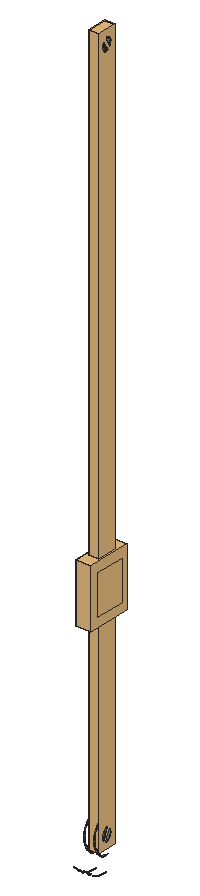
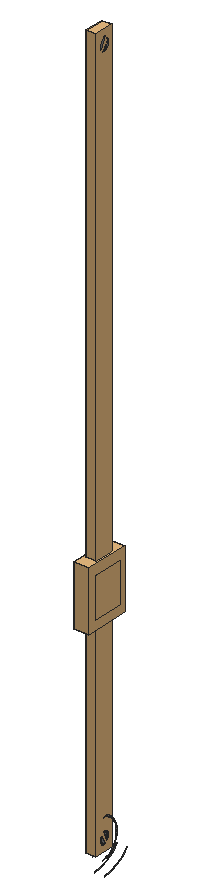
# SketchUp Ruby script. Lengths in inches.
U = 1.inch
M = Sketchup.active_model
def pt(a) = Geom::Point3d.new(a.map { |v| v * U })
def face(e, loops, mat)
  f = e.add_face(loops[0].map { |a| pt(a) })
  loops[1..].each { |l| e.add_face(l.map { |a| pt(a) }).erase! }
  f.material = f.back_material = mat if mat
  f
end
# faces: each face lists its corners as indices into pts; further lists are holes
def faces(e, pts, list, mat = nil) = list.each { |f| face(e, (f[0].is_a?(Array) ? f : [f]).map { |l| l.map { |i| pts[i] } }, mat) }
# xy, xz, yz: faces in a plane at the given z, y or x. An outline is a flat list of corners, or four numbers for a rectangle; further outlines are holes
def ring(l) = l.size == 4 ? [[l[0], l[1]], [l[2], l[1]], [l[2], l[3]], [l[0], l[3]]] : l.each_slice(2).to_a
def flat(e, list, mat, &to3) = list.each { |f| face(e, (f[0].is_a?(Array) ? f : [f]).map { |l| ring(l).map { |u, v| to3.(u, v) } }, mat) }
def xy(e, z, list, mat = nil) = flat(e, list, mat) { |x, y| [x, y, z] }
def xz(e, y, list, mat = nil) = flat(e, list, mat) { |x, z| [x, y, z] }
def yz(e, x, list, mat = nil) = flat(e, list, mat) { |y, z| [x, y, z] }
def lines(e, pts, list) = list.each { |a, b| e.add_line(pt(pts[a]), pt(pts[b])) }
# prism: a flat outline (further loops are holes) pulled along v
def prism(e, loops, v, mat = nil)
  f = face(e, loops, mat); d = Geom::Vector3d.new(v.map { |x| x * U })
  f.pushpull(f.normal.samedirection?(d) ? d.length : -d.length)
end
def box(e, o, s, mat = nil) = prism(e, [[o, [o[0] + s[0], o[1], o[2]], [o[0] + s[0], o[1] + s[1], o[2]], [o[0], o[1] + s[1], o[2]]]], [0, 0, s[2]], mat)
def at(x, y, z, deg = 0) = Geom::Transformation.translation(pt([x, y, z])) * Geom::Transformation.rotation(ORIGIN, Z_AXIS, deg.degrees)
def axes(o, x, y, z) = Geom::Transformation.new([*x, 0, *y, 0, *z, 0, *pt(o).to_a, 1])
def part(name) = M.definitions.add(name)
# library, detail: a bought-in or finely detailed component or shape, given as its bounding box
def library(name, o, s) = part(name).tap { |d| box(d.entities, o, s) }
def detail(e, o, s) = box(e.add_group.entities, o, s)
def put(e, d, t, mat = nil) = e.add_instance(d, t).tap { |i| i.material = mat if mat }
def group(e, t, mat = nil) = e.add_group.tap { |g| g.transformation = t; g.material = mat if mat }.entities
root = M.entities
M.materials.add("Material \#1").color = [140, 140, 140]
c1 = library("3DGeom~4_Defintion",[-18.02,-499.97,-221.16],[36.04,1000,262.12])
c2 = part("3DGeom~5_Defintion")
xy(c2.entities,-225.24,[[-0.79,-499.98,-2.33,-499.64,7.45,-496.14],[-0.79,-499.98,7.45,-496.14,1.58,-499.88],[1.58,-499.88,7.45,-496.14,3.84,-499.16],[-2.33,-499.64,7.4,-485.75,7.45,-496.14],[3.84,-499.16,7.45,-496.14,5.85,-497.89],
  [7.45,-496.14,7.4,-485.75,8.24,-487.08],[7.45,-496.14,8.24,-487.08,8.96,-489.34],[7.45,-496.14,8.96,-489.34,9.0625,-491.71],[7.45,-496.14,9.0625,-491.71,8.55,-494.03],[-7.4,-496.08,-8.24,-494.76,2.32,-482.2],
  [-8.24,-494.76,-8.96,-492.5,2.32,-482.2],[-8.96,-492.5,-9.0625,-490.125,2.32,-482.2],[-9.0625,-490.125,-8.55,-487.81,2.32,-482.2],[-8.55,-487.81,-7.45,-485.7,2.32,-482.2],[-7.45,-485.7,-5.85,-483.95,2.32,-482.2],
  [-5.85,-483.95,-3.84,-482.68,2.32,-482.2],[-3.84,-482.68,-1.58,-481.96,2.32,-482.2],[2.32,-482.2,-1.58,-481.96,0.79,-481.86],[0,481.82,-2.35,482.13,-6.92,496.71],[0,481.82,-6.92,496.71,1.55,482.04],
  [-2.35,482.13,-4.55,483.04,-6.92,496.71],[-4.55,483.04,-6.43,484.49,-6.92,496.71],[-6.43,484.49,-7.88,486.37,-6.92,496.71],[6.92,485.12,-1.55,499.8125,7.88,495.47],[6.92,485.12,7.88,495.47,7.88,486.37],
  [-7.88,486.37,-8.79,488.57,-6.92,496.71],[7.88,486.37,7.88,495.47,8.79,488.57],[-8.79,488.57,-9.1,490.92,-6.92,496.71],[8.79,488.57,7.88,495.47,9.1,490.92],[-9.1,490.92,-8.79,493.28,-6.92,496.71],
  [9.1,490.92,7.88,495.47,8.79,493.28],[-8.79,493.28,-7.88,495.47,-6.92,496.71],[7.88,495.47,-1.55,499.8125,0,500.02],[7.88,495.47,0,500.02,2.35,499.71],[7.88,495.47,2.35,499.71,4.55,498.8],
  [7.88,495.47,4.55,498.8,6.43,497.35]],"Material \#1")
xy(c2.entities,-221.57,[[-2.33,-499.64,-5.22,-498.37,7.4,-485.75],[-5.22,-498.37,-7.4,-496.08,5.22,-483.47],[-5.22,-498.37,5.22,-483.47,7.4,-485.75],[-7.4,-496.08,2.32,-482.2,5.22,-483.47],[1.55,482.04,-6.92,496.71,-4.55,498.8],
  [1.55,482.04,-4.55,498.8,4.55,483.04],[4.55,483.04,-4.55,498.8,-1.55,499.8125],[4.55,483.04,-1.55,499.8125,6.92,485.12]],"Material \#1")
xy(c2.entities,38.05,[[-2.33,-499.64,7.4,-485.75,-5.22,-498.37],[-5.22,-498.37,5.22,-483.47,-7.4,-496.08],[-5.22,-498.37,7.4,-485.75,5.22,-483.47],[-7.4,-496.08,5.22,-483.47,2.32,-482.2],[1.55,482.04,-4.55,498.8,-6.92,496.71],
  [1.55,482.04,4.55,483.04,-4.55,498.8],[4.55,483.04,-1.55,499.8125,-4.55,498.8],[4.55,483.04,6.92,485.12,-1.55,499.8125]],"Material \#1")
xy(c2.entities,41.72,[[-0.79,-499.98,7.45,-496.14,-2.33,-499.64],[-0.79,-499.98,1.58,-499.88,7.45,-496.14],[1.58,-499.88,3.84,-499.16,7.45,-496.14],[-2.33,-499.64,7.45,-496.14,7.4,-485.75],[3.84,-499.16,5.85,-497.89,7.45,-496.14],
  [7.45,-496.14,8.24,-487.08,7.4,-485.75],[7.45,-496.14,8.55,-494.03,9.0625,-491.71],[7.45,-496.14,8.96,-489.34,8.24,-487.08],[7.45,-496.14,9.0625,-491.71,8.96,-489.34],[-7.4,-496.08,2.32,-482.2,-8.24,-494.76],
  [-8.24,-494.76,2.32,-482.2,-8.96,-492.5],[-8.96,-492.5,2.32,-482.2,-9.0625,-490.125],[-9.0625,-490.125,2.32,-482.2,-8.55,-487.81],[-8.55,-487.81,2.32,-482.2,-7.45,-485.7],[-7.45,-485.7,2.32,-482.2,-5.85,-483.95],
  [-5.85,-483.95,2.32,-482.2,-3.84,-482.68],[-3.84,-482.68,2.32,-482.2,-1.58,-481.96],[2.32,-482.2,0.79,-481.86,-1.58,-481.96],[0,481.82,-6.92,496.71,-2.35,482.13],[0,481.82,1.55,482.04,-6.92,496.71],
  [-2.35,482.13,-6.92,496.71,-4.55,483.04],[-4.55,483.04,-6.92,496.71,-6.43,484.49],[-6.43,484.49,-6.92,496.71,-7.88,486.37],[6.92,485.12,7.88,495.47,-1.55,499.8125],[6.92,485.12,7.88,486.37,7.88,495.47],
  [-7.88,486.37,-6.92,496.71,-8.79,488.57],[7.88,486.37,8.79,488.57,7.88,495.47],[-8.79,488.57,-6.92,496.71,-9.1,490.92],[8.79,488.57,9.1,490.92,7.88,495.47],[-9.1,490.92,-6.92,496.71,-8.79,493.28],
  [9.1,490.92,8.79,493.28,7.88,495.47],[-8.79,493.28,-6.92,496.71,-7.88,495.47],[7.88,495.47,0,500.02,-1.55,499.8125],[7.88,495.47,2.35,499.71,0,500.02],[7.88,495.47,4.55,498.8,2.35,499.71],
  [7.88,495.47,6.43,497.35,4.55,498.8]],"Material \#1")
c3 = library("3DGeom~14_Defintion",[-102.17,352.37,-727.27],[204.35,204.35,1000])
c4 = library("3DGeom~1_Defintion",[-60.87,347.29,-704.08],[121.74,121.75,1000])
yz(root,263.952,[[328.177,50.586,328.059,50.6,328.061,50.614],[328.177,50.586,328.061,50.614,328.177,50.601],[328.059,50.6,327.948,50.64,327.952,50.654],[328.059,50.6,327.952,50.654,328.061,50.614],[327.948,50.64,327.846,50.704,327.852,50.717],
  [327.948,50.64,327.852,50.717,327.952,50.654],[327.846,50.704,327.762,50.801,327.852,50.717],[328.177,50.818,328.138,50.822,328.14,50.837],[328.177,50.818,328.14,50.837,328.177,50.832],[328.177,50.818,328.177,50.832,328.216,50.822],
  [328.138,50.822,328.101,50.836,328.105,50.85],[328.138,50.822,328.105,50.85,328.14,50.837],[328.101,50.836,328.067,50.857,328.073,50.87],[328.101,50.836,328.073,50.87,328.105,50.85],[328.067,50.857,328.037,50.885,328.044,50.897],
  [328.067,50.857,328.044,50.897,328.073,50.87],[328.037,50.885,328.011,50.92,328.019,50.93],[328.037,50.885,328.019,50.93,328.044,50.897],[328.011,50.92,327.989,50.96,327.999,50.968],[328.011,50.92,327.999,50.968,328.019,50.93],
  [327.989,50.96,327.973,51.005,327.984,51.01],[327.989,50.96,327.984,51.01,327.999,50.968],[327.973,51.005,327.963,51.054,327.974,51.057],[327.973,51.005,327.974,51.057,327.984,51.01],[327.963,51.054,327.959,51.092,327.971,51.092],
  [327.963,51.054,327.971,51.092,327.974,51.057],[327.959,51.092,327.963,51.157,327.974,51.154],[327.959,51.092,327.974,51.154,327.971,51.092],[327.974,51.154,327.963,51.157,327.984,51.201],[327.963,51.157,327.973,51.206,327.984,51.201],
  [327.984,51.201,327.973,51.206,327.999,51.243],[327.973,51.206,327.989,51.251,327.999,51.243],[327.999,51.243,327.989,51.251,328.019,51.281],[327.989,51.251,328.011,51.291,328.019,51.281],[328.019,51.281,328.011,51.291,328.044,51.314],
  [328.011,51.291,328.037,51.325,328.044,51.314],[328.044,51.314,328.037,51.325,328.073,51.341],[328.037,51.325,328.067,51.354,328.073,51.341],[328.073,51.341,328.067,51.354,328.105,51.361],[328.067,51.354,328.101,51.375,328.105,51.361],
  [328.105,51.361,328.101,51.375,328.14,51.374],[328.14,51.374,328.101,51.375,328.138,51.389],[328.14,51.374,328.138,51.389,328.177,51.378],[328.214,51.374,328.177,51.378,328.177,51.393],[328.177,51.378,328.138,51.389,328.177,51.393]],"Material \#1")
yz(root,264.101,[[328.177,50.586,328.061,50.614,328.059,50.6],[328.177,50.586,328.177,50.601,328.061,50.614],[328.059,50.6,327.952,50.654,327.948,50.64],[328.059,50.6,328.061,50.614,327.952,50.654],[327.948,50.64,327.852,50.717,327.846,50.704],
  [327.948,50.64,327.952,50.654,327.852,50.717],[327.846,50.704,327.852,50.717,327.762,50.801],[328.177,50.818,328.14,50.837,328.138,50.822],[328.177,50.818,328.177,50.832,328.14,50.837],[328.177,50.818,328.216,50.822,328.177,50.832],
  [328.138,50.822,328.105,50.85,328.101,50.836],[328.138,50.822,328.14,50.837,328.105,50.85],[328.101,50.836,328.073,50.87,328.067,50.857],[328.101,50.836,328.105,50.85,328.073,50.87],[328.067,50.857,328.044,50.897,328.037,50.885],
  [328.067,50.857,328.073,50.87,328.044,50.897],[328.037,50.885,328.019,50.93,328.011,50.92],[328.037,50.885,328.044,50.897,328.019,50.93],[328.011,50.92,327.999,50.968,327.989,50.96],[328.011,50.92,328.019,50.93,327.999,50.968],
  [327.989,50.96,327.984,51.01,327.973,51.005],[327.989,50.96,327.999,50.968,327.984,51.01],[327.973,51.005,327.974,51.057,327.963,51.054],[327.973,51.005,327.984,51.01,327.974,51.057],[327.963,51.054,327.971,51.092,327.959,51.092],
  [327.963,51.054,327.974,51.057,327.971,51.092],[327.959,51.092,327.971,51.092,327.974,51.154],[327.959,51.092,327.974,51.154,327.963,51.157],[327.974,51.154,327.984,51.201,327.963,51.157],[327.963,51.157,327.984,51.201,327.973,51.206],
  [327.984,51.201,327.999,51.243,327.973,51.206],[327.973,51.206,327.999,51.243,327.989,51.251],[327.999,51.243,328.019,51.281,327.989,51.251],[327.989,51.251,328.019,51.281,328.011,51.291],[328.019,51.281,328.044,51.314,328.011,51.291],
  [328.011,51.291,328.044,51.314,328.037,51.325],[328.044,51.314,328.073,51.341,328.037,51.325],[328.037,51.325,328.073,51.341,328.067,51.354],[328.073,51.341,328.105,51.361,328.067,51.354],[328.067,51.354,328.105,51.361,328.101,51.375],
  [328.105,51.361,328.14,51.374,328.101,51.375],[328.14,51.374,328.138,51.389,328.101,51.375],[328.14,51.374,328.177,51.378,328.138,51.389],[328.214,51.374,328.177,51.393,328.177,51.378],[328.177,51.378,328.177,51.393,328.138,51.389]],"Material \#1")
p = [[263.952,328.152,50.98],[263.953,328.138,50.947],[263.955,328.138,50.947],[263.954,328.152,50.98],[263.953,328.114,50.96],[263.955,328.114,50.96],
  [264.101,328.152,50.98],[264.099,328.152,50.98],[264.098,328.138,50.947],[264.1,328.138,50.947],[264.098,328.114,50.96],[264.1,328.114,50.96],
  [263.953,328.093,50.981],[263.955,328.093,50.981],[263.952,328.108,51.014],[263.954,328.108,51.014],[263.952,328.121,51.043],[263.954,328.121,51.043],
  [263.952,328.19,51.201],[263.954,328.19,51.201],[264.098,328.093,50.981],[264.1,328.093,50.981],[264.099,328.108,51.014],[264.101,328.108,51.014],
  [264.099,328.121,51.043],[264.101,328.121,51.043],[264.099,328.19,51.201],[264.101,328.19,51.201],[263.952,328.165,51.009],[263.954,328.164,51.009],
  [263.952,328.234,51.168],[263.954,328.234,51.168],[264.101,328.164,51.009],[264.099,328.164,51.009],[264.101,328.234,51.168],[264.099,328.234,51.168],
  [263.952,328.203,51.231],[263.954,328.203,51.231],[263.953,328.217,51.263],[263.955,328.217,51.263],[263.953,328.241,51.251],[263.953,328.261,51.23],
  [263.955,328.261,51.23],[263.955,328.241,51.251],[263.952,328.247,51.197],[263.954,328.247,51.197],[264.099,328.203,51.231],[264.101,328.203,51.231],
  [264.098,328.217,51.263],[264.1,328.217,51.263],[264.1,328.241,51.251],[264.098,328.241,51.251],[264.098,328.261,51.23],[264.1,328.261,51.23],
  [264.099,328.247,51.197],[264.101,328.247,51.197]]
faces(root,p,[[0,1,2],[2,3,0],[1,4,5],[5,2,1],[6,7,8],[8,9,6],[9,8,10],[10,11,9],
  [4,12,13],[13,5,4],[12,14,15],[15,13,12],[14,16,17],[17,15,14],[16,18,19],[19,17,16],
  [11,10,20],[20,21,11],[21,20,22],[22,23,21],[23,22,24],[24,25,23],[25,24,26],[26,27,25],
  [28,0,3],[3,29,28],[30,28,29],[29,31,30],[32,33,7],[7,6,32],[34,35,33],[33,32,34],
  [18,36,37],[37,19,18],[36,38,39],[39,37,36],[40,41,42],[42,43,40],[41,44,45],[45,42,41],
  [44,30,31],[31,45,44],[27,26,46],[46,47,27],[47,46,48],[48,49,47],[50,51,52],[52,53,50],
  [53,52,54],[54,55,53],[55,54,35],[35,34,55],[38,40,43],[43,39,38],[49,48,51],[51,50,49]],"Material \#1")
put(root,c1,axes([263.98,328.18,56.41],[0,0.00832,0],[0,0,-0.011],[-0.00057,0,0]),"Material \#1")
put(root,c2,axes([263.98,328.18,56.41],[0,0.00817,0],[0,0,-0.0108],[-0.00056,0,0]),"Material \#1")
put(root,c3,axes([263.98,328.18,56.41],[0,0.0033,0],[0,0,-0.00436],[-0.00023,0,0]),"Material \#1")
put(root,c4,axes([263.98,328.18,56.41],[0,0.00367,0],[0,0,-0.00485],[-0.00025,0,0]),"Material \#1")
